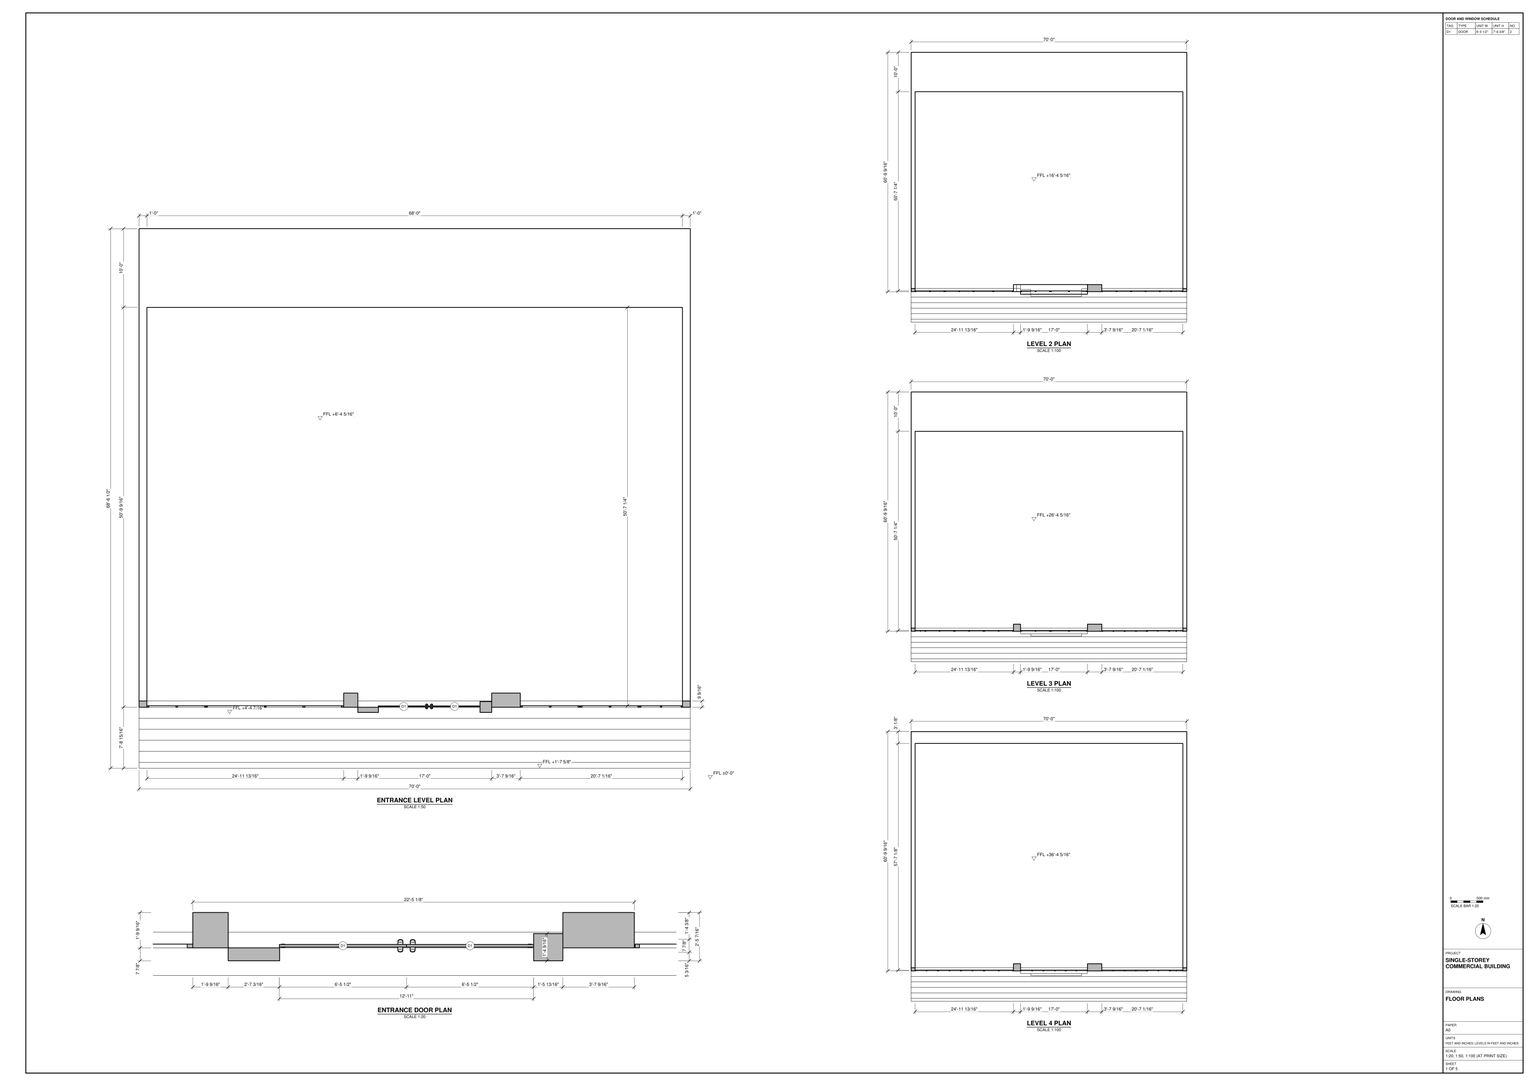
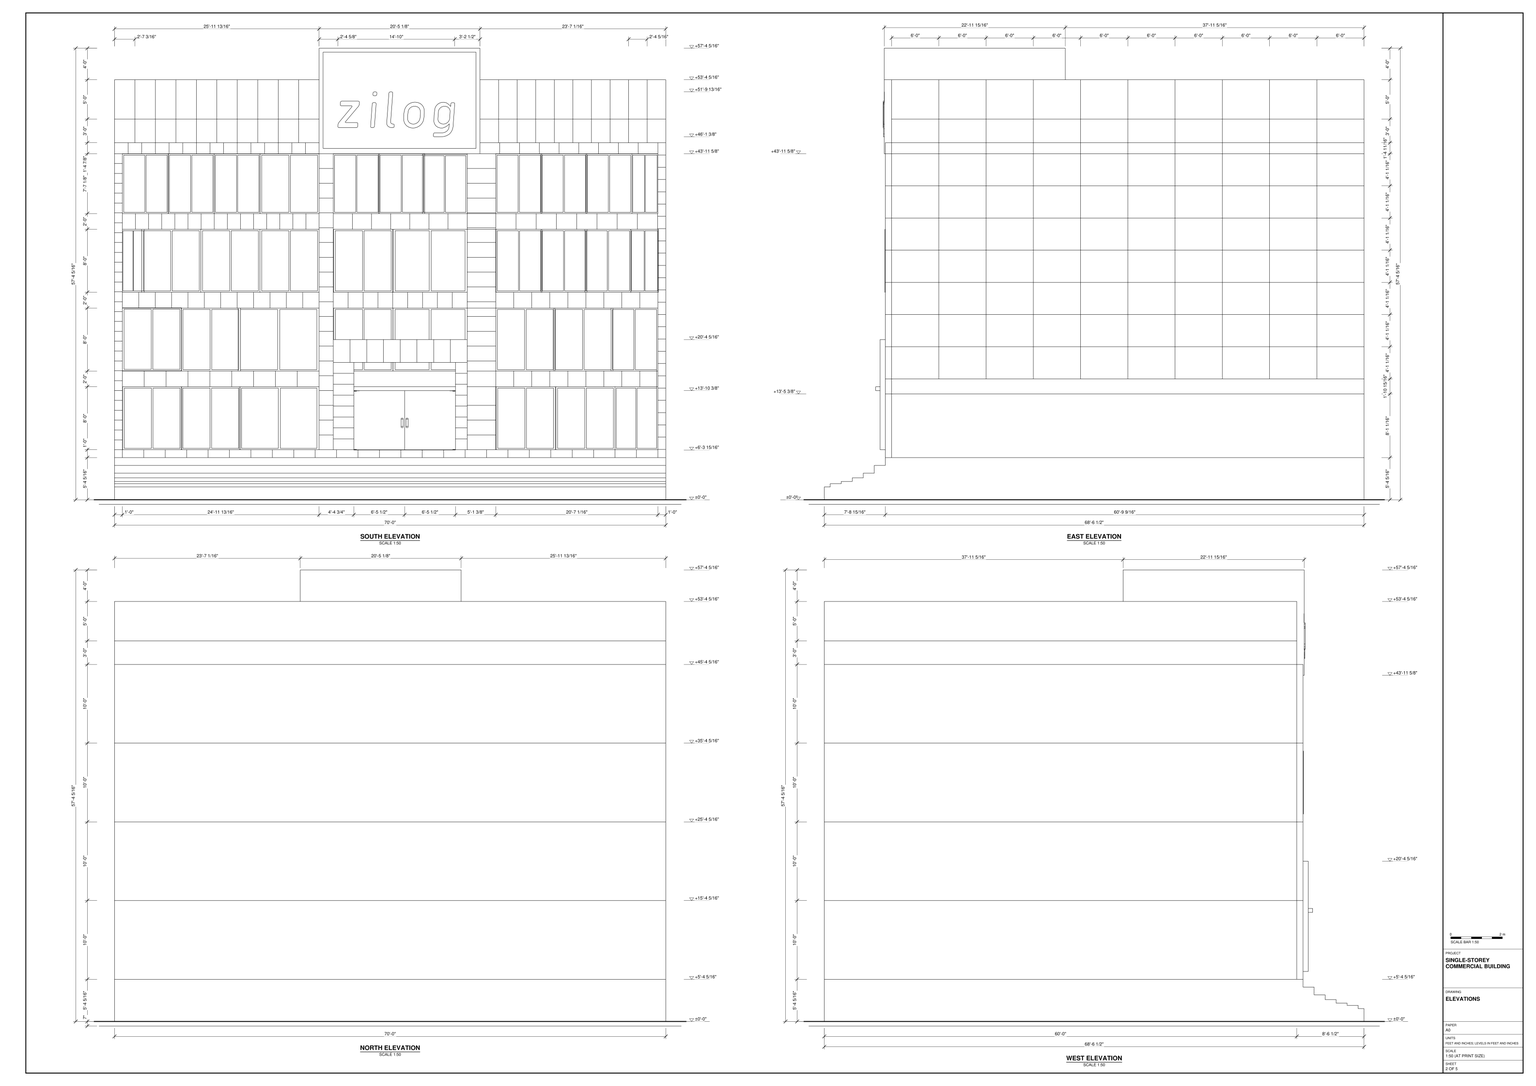
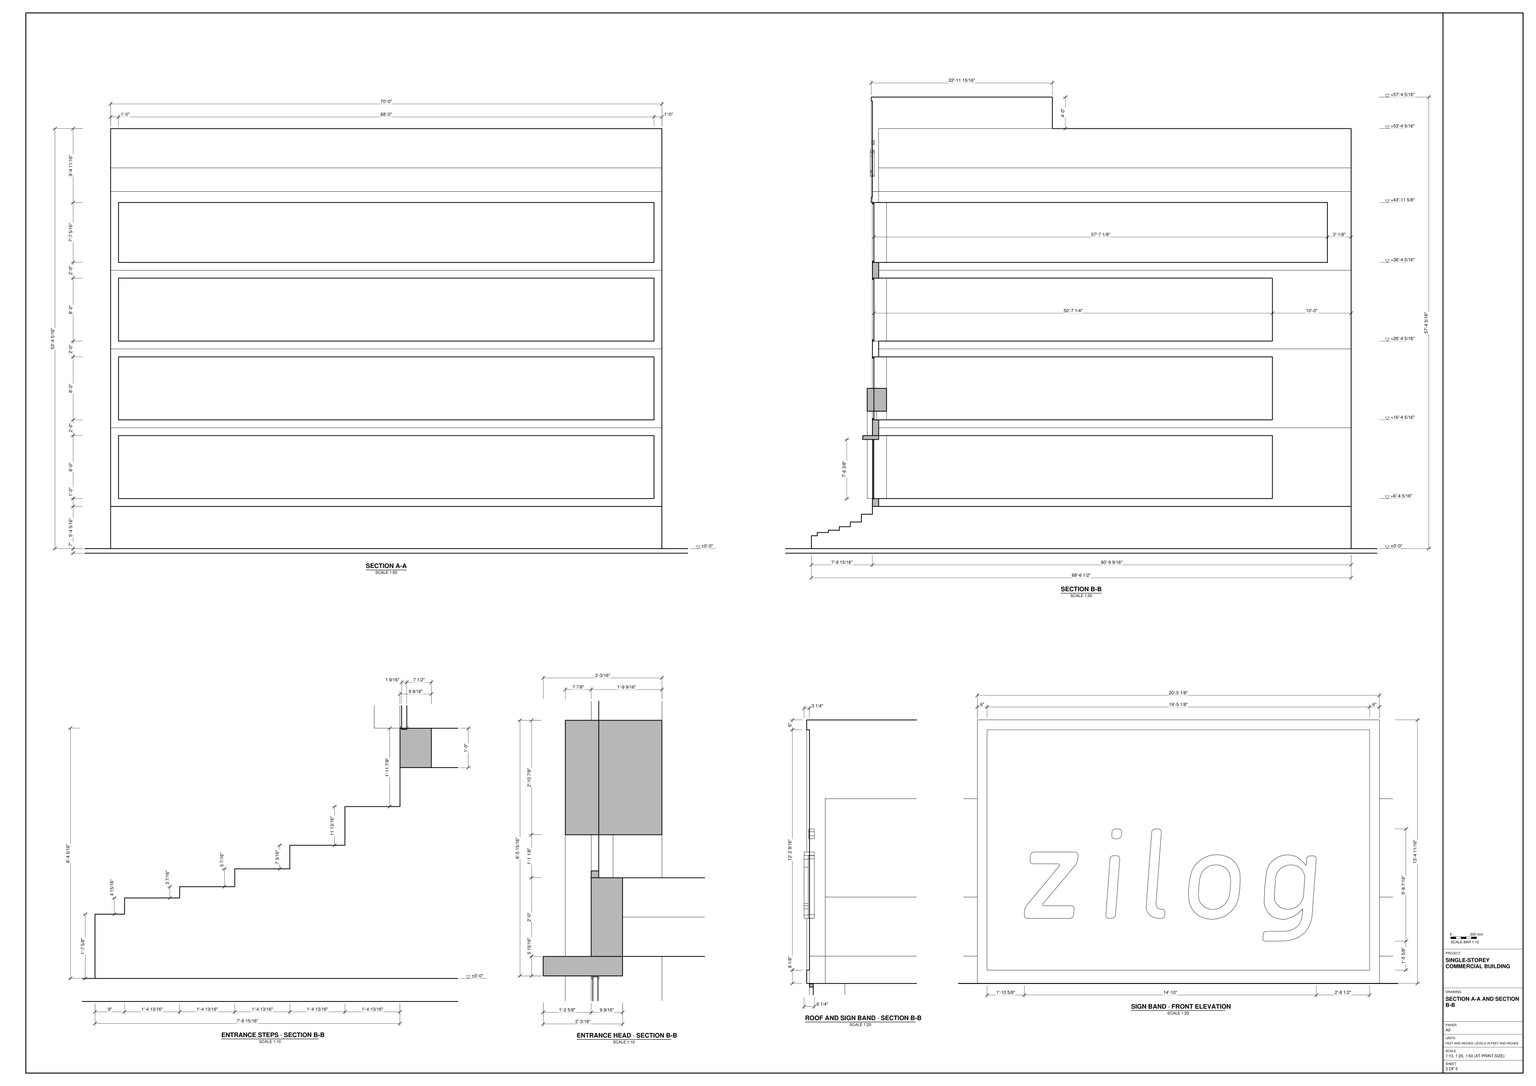
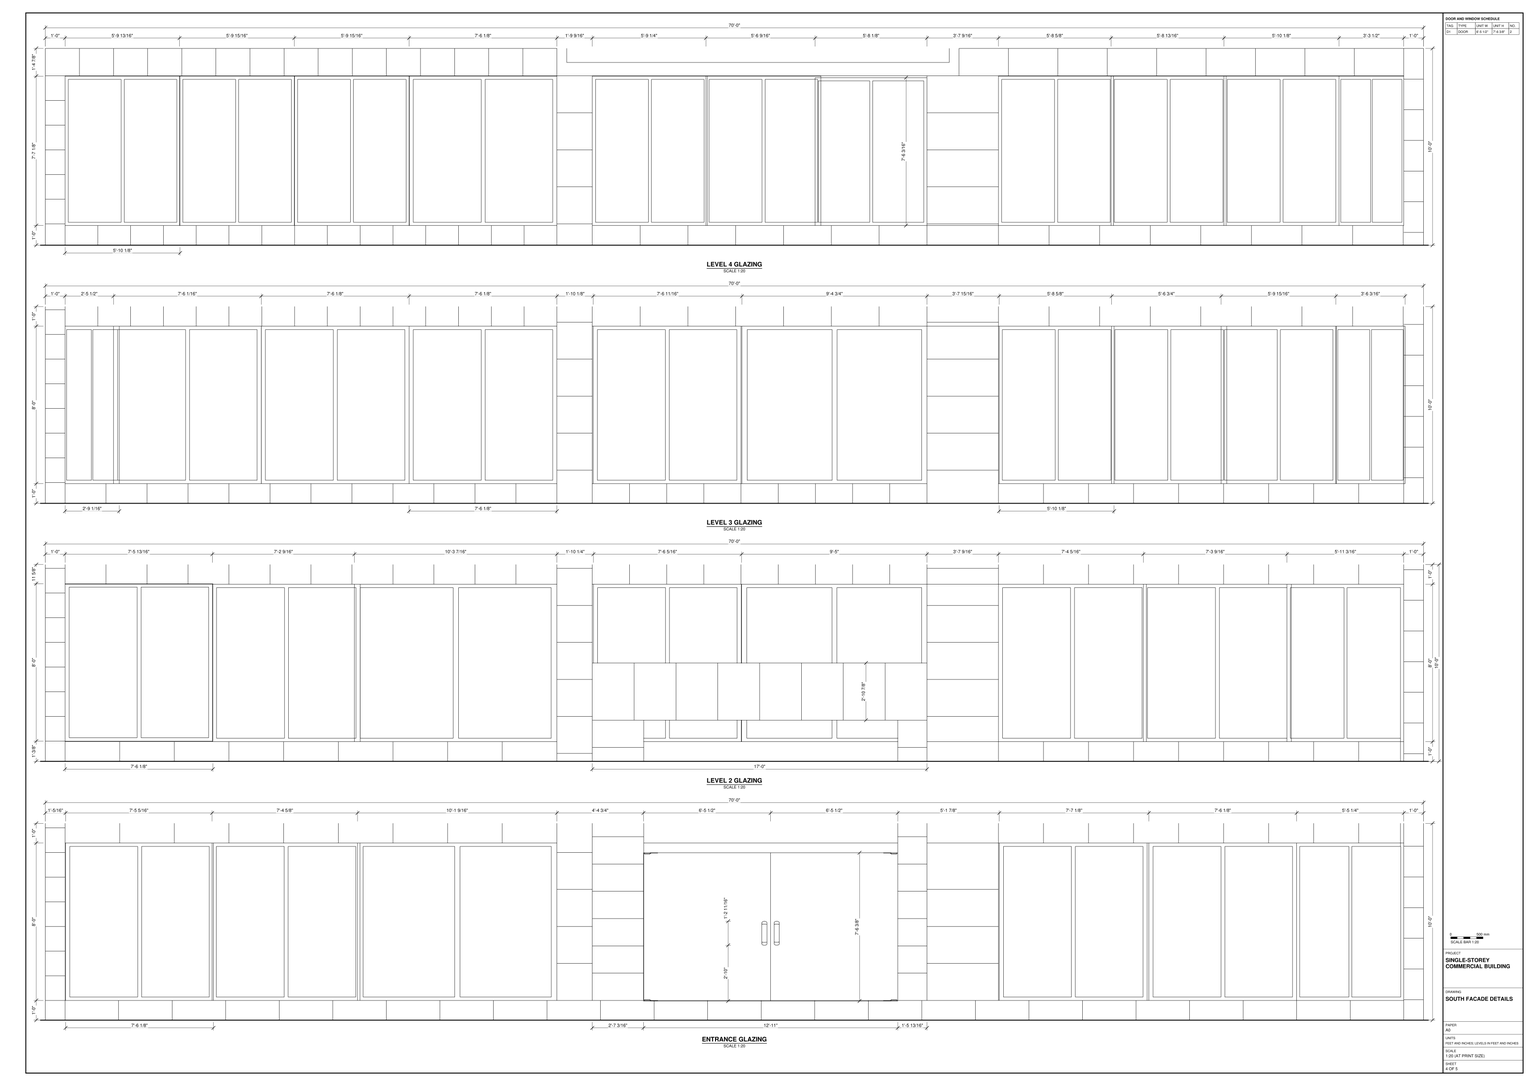
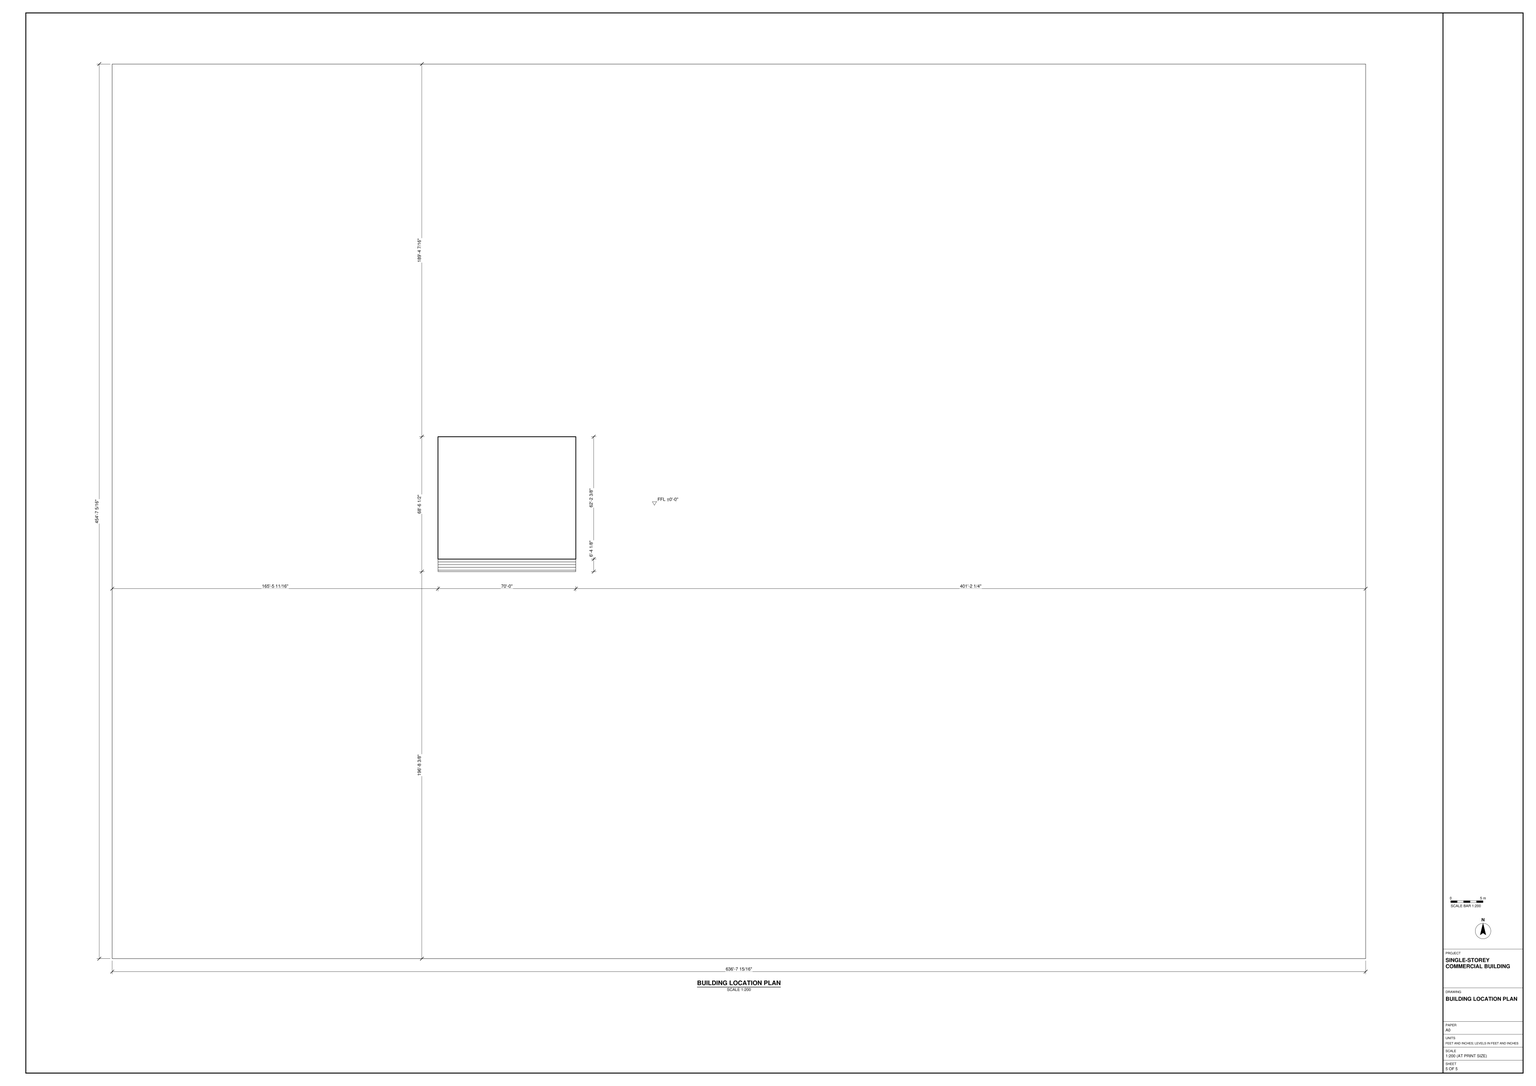
Build the commercial building in SketchUp from task_files/diagram_01.pdf. Work in feet and inches. The overall model extents are 636'-7 15/16" along X, 454'-7 5/16" along Y and 57'-11 5/16" along Z. These are the extents of the whole model; use the dimensioned plans for the building footprint. Set the ground datum at ±0'-0" and use the plans and sections to position the raised entrance floor and the three floors above it.

Model the rectangular shell with the wall and slab thicknesses shown in section. Keep the floor areas open and carry the uppermost floor space farther towards the rear than the spaces below it. Run the entrance steps across the south frontage to the paired glass doors. Use the entrance details to form the jambs and projecting head. Lay out the south window units in bays, matching the mullions and the bands between rows to the elevation. Distinguish the panel grid on the east wall from the horizontal divisions on the north and west walls. Finish the flat roof with the raised, framed sign panel above the entrance bay.

Make the walls, slabs and roof separate groups or components, and keep each furniture or joinery piece separate in the same way. Use components for repeated parts such as window units. Any decor or loose items shown may be represented by suitable library components. Save one SketchUp model as output_files/commercial_building_with_stepped_entrance_and_sign_band.skp.

# SketchUp Ruby script. Lengths in inches.
U = 1.inch
M = Sketchup.active_model
def pt(a) = Geom::Point3d.new(a.map { |v| v * U })
def face(e, loops, mat)
  f = e.add_face(loops[0].map { |a| pt(a) })
  loops[1..].each { |l| e.add_face(l.map { |a| pt(a) }).erase! }
  f.material = f.back_material = mat if mat
  f
end
# faces: each face lists its corners as indices into pts; further lists are holes
def faces(e, pts, list, mat = nil) = list.each { |f| face(e, (f[0].is_a?(Array) ? f : [f]).map { |l| l.map { |i| pts[i] } }, mat) }
# xy, xz, yz: faces in a plane at the given z, y or x. An outline is a flat list of corners, or four numbers for a rectangle; further outlines are holes
def ring(l) = l.size == 4 ? [[l[0], l[1]], [l[2], l[1]], [l[2], l[3]], [l[0], l[3]]] : l.each_slice(2).to_a
def flat(e, list, mat, &to3) = list.each { |f| face(e, (f[0].is_a?(Array) ? f : [f]).map { |l| ring(l).map { |u, v| to3.(u, v) } }, mat) }
def xy(e, z, list, mat = nil) = flat(e, list, mat) { |x, y| [x, y, z] }
def xz(e, y, list, mat = nil) = flat(e, list, mat) { |x, z| [x, y, z] }
def yz(e, x, list, mat = nil) = flat(e, list, mat) { |y, z| [x, y, z] }
def lines(e, pts, list) = list.each { |a, b| e.add_line(pt(pts[a]), pt(pts[b])) }
# prism: a flat outline (further loops are holes) pulled along v
def prism(e, loops, v, mat = nil)
  f = face(e, loops, mat); d = Geom::Vector3d.new(v.map { |x| x * U })
  f.pushpull(f.normal.samedirection?(d) ? d.length : -d.length)
end
def box(e, o, s, mat = nil) = prism(e, [[o, [o[0] + s[0], o[1], o[2]], [o[0] + s[0], o[1] + s[1], o[2]], [o[0], o[1] + s[1], o[2]]]], [0, 0, s[2]], mat)
def at(x, y, z, deg = 0) = Geom::Transformation.translation(pt([x, y, z])) * Geom::Transformation.rotation(ORIGIN, Z_AXIS, deg.degrees)
def axes(o, x, y, z) = Geom::Transformation.new([*x, 0, *y, 0, *z, 0, *pt(o).to_a, 1])
def part(name) = M.definitions.add(name)
# library, detail: a bought-in or finely detailed component or shape, given as its bounding box
def library(name, o, s) = part(name).tap { |d| box(d.entities, o, s) }
def detail(e, o, s) = box(e.add_group.entities, o, s)
def put(e, d, t, mat = nil) = e.add_instance(d, t).tap { |i| i.material = mat if mat }
def group(e, t, mat = nil) = e.add_group.tap { |g| g.transformation = t; g.material = mat if mat }.entities
root = M.entities
M.materials.add("2").color = [128, 128, 128]
M.materials["2"].alpha = 0.5
M.materials.add("Teddy_Shoes").color = [189, 191, 193]
M.materials.add("[0079_Teal]").color = [0, 68, 68]
M.materials.add("[0102_RoyalBlue]").color = [32, 52, 112]
M.materials.add("[0132_LightGray]").color = [169, 169, 169]
M.materials.add("[0134_DimGray]").color = [105, 105, 105]
M.materials.add("[0135_DarkGray]").color = [81, 81, 81]
M.materials.add("[0137_Black]").color = [0, 0, 0]
c1 = part("WindowDoubleBlack")
xy(c1.entities,0,[[0,0,96.0625,1.57]],"[0137_Black]")
xy(c1.entities,2.71,[[2.71,0,46.85,1.57],[49.41,0,93.35,1.57]],"[0137_Black]")
xy(c1.entities,122.09,[[2.71,0,46.85,1.57],[49.41,0,50,1.57],[50,0,93.35,1.57]],"[0137_Black]")
xy(c1.entities,124.8,[[0,0,96.0625,1.57]],"[0137_Black]")
xz(c1.entities,0,[[[0,0,96.0625,124.8],[2.71,2.71,46.85,122.09],[49.41,2.71,93.35,122.09]]],"[0137_Black]")
xz(c1.entities,1.57,[[2.71,2.71,46.85,122.09],[49.41,2.71,93.35,122.09]],"2")
xz(c1.entities,1.57,[[[0,0,96.0625,124.8],[2.71,2.71,46.85,122.09],[49.41,2.71,93.35,122.09]]],"[0137_Black]")
yz(c1.entities,0,[[0,0,1.57,124.8]],"[0137_Black]")
yz(c1.entities,2.71,[[0,2.71,1.57,122.09]],"[0137_Black]")
yz(c1.entities,46.85,[[0,2.71,1.57,122.09]],"[0137_Black]")
yz(c1.entities,49.41,[[0,2.71,1.57,122.09]],"[0137_Black]")
yz(c1.entities,93.35,[[0,2.71,1.57,122.09]],"[0137_Black]")
yz(c1.entities,96.0625,[[0,0,1.57,124.8]],"[0137_Black]")
c2 = library("Glass_door",[70.54,1.5625,0],[78.74,7.87,82.68])
c3 = library("Group\#1",[0,0,0],[237.3,8.35,91.24])
c4 = part("zilog")
put(c4.entities,c3,at(0,150.05,41.16))
xy(root,-25.25,[[0,0,7639.9375,5455.3125]])
xy(root,-18.22,[[[0,0,7639.9375,5455.3125],[1985.6875,2360.375,2825.6875,3182.875]],[1985.6875,2360.375,2825.6875,3182.875]])
xy(root,1.375,[[1985.6875,2360.375,2825.6875,2369.375]])
xy(root,6.3125,[[1985.6875,2369.375,2825.6875,2386.16]])
xy(root,9.75,[[1985.6875,2386.16,2825.6875,2402.95]])
xy(root,15.1875,[[1985.6875,2402.95,2825.6875,2419.74]])
xy(root,22.375,[[1985.6875,2419.74,2825.6875,2436.52]])
xy(root,34.1875,[[1985.6875,2436.52,2825.6875,2453.3125]])
xy(root,46.0625,[[1985.6875,2453.3125,2825.6875,2462.875],[1985.6875,2462.875,2825.6875,3182.875]],"[0102_RoyalBlue]")
xy(root,58.0625,[[2319.0625,2445.4375,2350.4375,2453.3125],[2505.24,2445.4375,2523.05,2453.3125],[1997.6875,2453.3125,2297.5,2462.875],[2297.5,2453.3125,2319.0625,2462.875],[2319.0625,2453.3125,2505.24,2453.3125,2505.24,2462,2523.05,2462,2523.05,2462.875,2319.0625,2462.875],
  [2505.24,2453.3125,2523.05,2462],[2523.05,2453.3125,2566.625,2462.875],[2566.625,2453.3125,2813.6875,2462.875],[1997.6875,2462.875,2297.5,2462.875,2297.5,2474.875,2319.0625,2474.875,2319.0625,2462.875,2523.05,2462.875,2523.05,2474.875,2566.625,2474.875,2566.625,2462.875,2813.6875,2462.875,2813.6875,3062.875,1997.6875,3062.875],[2297.5,2462.875,2319.0625,2474.875],
  [2523.05,2462.875,2566.625,2474.875]],"[0102_RoyalBlue]")
xy(root,148.125,[[2350.4375,2438.6875,2350.4375,2453.3125,2319.0625,2453.3125,2319.0625,2462.875,2505.24,2462.875,2505.24,2438.6875]],"[0102_RoyalBlue]")
xy(root,154.0625,[[2350.4375,2438.6875,2505.24,2453.3125],[1997.6875,2453.3125,2297.5,2462.875],[2319.0625,2453.3125,2505.24,2462.875],[2505.24,2453.3125,2813.6875,2462.875],[1997.6875,2462.875,1997.6875,3062.875,2813.6875,3062.875,2813.6875,2462.875,2566.625,2462.875,2566.625,2474.875,2523.05,2474.875,2523.05,2462.875,2319.0625,2462.875,2319.0625,2474.875,2297.5,2474.875,2297.5,2462.875],
  [2297.5,2462.875,2307.0625,2474.875],[2307.0625,2462.875,2319.0625,2474.875],[2523.05,2462.875,2566.625,2474.875]],"[0102_RoyalBlue]")
xy(root,178.0625,[[1997.6875,2453.3125,2297.5,2462.875],[2319.0625,2453.3125,2350.4375,2459.9375],[2350.4375,2453.3125,2813.6875,2453.3125,2813.6875,2462.875,2319.0625,2462.875,2319.0625,2459.9375,2350.4375,2459.9375],[1997.6875,2462.875,2297.5,2462.875,2297.5,2474.875,2319.0625,2474.875,2319.0625,2462.875,2523.05,2462.875,2523.05,2474.875,2566.625,2474.875,2566.625,2462.875,2813.6875,2462.875,2813.6875,3062.875,1997.6875,3062.875],[2297.5,2462.875,2307.0625,2474.875],
  [2307.0625,2462.875,2319.0625,2474.875],[2523.05,2462.875,2566.625,2474.875]],"[0102_RoyalBlue]")
xy(root,191.17,[[2350.4375,2445.4375,2350.4375,2459.9375,2319.0625,2459.9375,2319.0625,2474.875,2523.05,2474.875,2523.05,2462,2505.24,2462,2505.24,2445.4375]],"[0102_RoyalBlue]")
xy(root,226.0625,[[2319.0625,2445.4375,2523.05,2474.875]],"[0134_DimGray]")
xy(root,274.0625,[[1997.6875,2453.3125,2297.5,2462.875],[2319.0625,2453.3125,2813.6875,2462.875],[1997.6875,2462.875,1997.6875,3062.875,2813.6875,3062.875,2813.6875,2462.875,2566.625,2462.875,2566.625,2474.875,2523.05,2474.875,2523.05,2462.875,2319.0625,2462.875,2319.0625,2474.875,2297.5,2474.875,2297.5,2462.875],[2297.5,2462.875,2307.0625,2474.875],[2307.0625,2462.875,2319.0625,2474.875],
  [2523.05,2462.875,2566.625,2474.875]],"[0102_RoyalBlue]")
xy(root,298.0625,[[1997.6875,2453.3125,2297.5,2462.875],[1997.6875,2462.875,2297.5,2462.875,2297.5,2474.875,2319.0625,2474.875,2319.0625,2462.875,2523.05,2462.875,2523.05,2474.875,2566.625,2474.875,2566.625,2462.875,2813.6875,2462.875,2813.6875,3062.875,1997.6875,3062.875],[2297.5,2462.875,2307.0625,2474.875],[2307.0625,2462.875,2319.0625,2474.875],[2523.05,2462.875,2566.625,2474.875]],"[0102_RoyalBlue]")
xy(root,394.0625,[[1997.6875,2453.3125,2297.5,2462.875],[2319.0625,2453.3125,2813.6875,2462.875],[1997.6875,2462.875,1997.6875,3062.875,2813.6875,3062.875,2813.6875,2462.875,2566.625,2462.875,2566.625,2474.875,2523.05,2474.875,2523.05,2462.875,2319.0625,2462.875,2319.0625,2474.875,2297.5,2474.875,2297.5,2462.875],[2297.5,2462.875,2307.0625,2474.875],[2307.0625,2462.875,2319.0625,2474.875],
  [2523.05,2462.875,2566.625,2474.875]],"[0102_RoyalBlue]")
xy(root,418.0625,[[1997.6875,2453.3125,2297.5,2462.875],[2319.0625,2453.3125,2813.6875,2462.875],[1997.6875,2462.875,2297.5,2462.875,2297.5,2474.875,2319.0625,2474.875,2319.0625,2462.875,2523.05,2462.875,2523.05,2474.875,2566.625,2474.875,2566.625,2462.875,2813.6875,2462.875,2813.6875,3146.75,1997.6875,3146.75],[2297.5,2462.875,2307.0625,2474.875],[2307.0625,2462.875,2319.0625,2474.875],
  [2523.05,2462.875,2566.625,2474.875]],"[0102_RoyalBlue]")
xy(root,509.375,[[2297.5,2451.625,2542.625,2453.3125],[1997.6875,2453.3125,2297.5,2462.875],[2297.5,2453.3125,2319.0625,2474.875],[2319.0625,2453.3125,2523.05,2462.875],[2523.05,2453.3125,2542.625,2474.875],
  [2542.625,2453.3125,2566.625,2462.875],[2566.625,2453.3125,2813.6875,2462.875],[1997.6875,2462.875,1997.6875,3146.75,2813.6875,3146.75,2813.6875,2462.875,2566.625,2462.875,2566.625,2474.875,2523.05,2474.875,2523.05,2462.875,2319.0625,2462.875,2319.0625,2474.875,2297.5,2474.875,2297.5,2462.875],[2542.625,2462.875,2566.625,2474.875]],"[0102_RoyalBlue]")
xy(root,517.5,[[2303.5,2451.625,2536.625,2453.3125]],"[0102_RoyalBlue]")
xy(root,526.0625,[[1985.6875,2453.3125,2297.5,2462.875],[2542.625,2453.3125,2825.6875,2462.875]],"[0102_RoyalBlue]")
xy(root,622.0625,[[1985.6875,2462.875,2297.5,3182.875],[2542.625,2462.875,2825.6875,3182.875],[2297.5,2727.59,2542.625,3182.875]],"[0102_RoyalBlue]")
xy(root,664.0625,[[2303.5,2451.625,2536.625,2453.3125]])
xy(root,670.0625,[[2297.5,2451.625,2542.625,2727.59]],"[0102_RoyalBlue]")
xz(root,0,[[0,-25.25,7639.9375,-18.22]])
xz(root,2360.375,[[1985.6875,-18.22,2825.6875,1.375]])
xz(root,2369.375,[[1985.6875,1.375,2825.6875,6.3125]])
xz(root,2386.16,[[1985.6875,6.3125,2825.6875,9.75]])
xz(root,2402.95,[[1985.6875,9.75,2825.6875,15.1875]])
xz(root,2419.74,[[1985.6875,15.1875,2825.6875,22.375]])
xz(root,2436.52,[[1985.6875,22.375,2825.6875,34.1875]])
xz(root,2438.6875,[[2350.4375,148.125,2505.24,154.0625]],"[0102_RoyalBlue]")
xz(root,2445.4375,[[2319.0625,58.0625,2350.4375,74.7],[2505.24,58.0625,2523.05,74.7],[2319.0625,74.7,2350.4375,91.34],[2505.24,74.7,2523.05,91.34],[2319.0625,91.34,2350.4375,107.98],
  [2505.24,91.34,2523.05,107.98],[2319.0625,107.98,2350.4375,124.62],[2505.24,107.98,2523.05,124.62],[2319.0625,124.62,2350.4375,141.26],[2505.24,124.62,2523.05,141.26],
  [2319.0625,141.26,2350.4375,157.9],[2505.24,141.26,2523.05,157.9],[2319.0625,157.9,2350.4375,174.53],[2505.24,157.9,2523.05,174.53],[2319.0625,174.53,2350.4375,191.17],
  [2505.24,174.53,2523.05,191.17],[2319.0625,191.17,2344.5625,226.0625],[2344.5625,191.17,2370.06,226.0625],[2370.06,191.17,2395.56,226.0625],[2395.56,191.17,2421.06,226.0625],
  [2421.06,191.17,2446.56,226.0625],[2446.56,191.17,2472.05,226.0625],[2472.05,191.17,2497.55,226.0625],[2497.55,191.17,2523.05,226.0625]],"[0134_DimGray]")
xz(root,2451.625,[[[2297.5,509.375,2542.625,670.0625],[2303.5,517.5,2536.625,664.0625]]],"[0102_RoyalBlue]")
xz(root,2453.3125,[[1985.6875,34.1875,2825.6875,46.0625]])
xz(root,2453.3125,[[2519.93,46.0625,2552.57,58.0625],[2552.57,46.0625,2585.21,58.0625],[2585.21,46.0625,2617.85,58.0625],[2617.85,46.0625,2650.49,58.0625],[2650.49,46.0625,2683.13,58.0625],
  [2683.13,46.0625,2715.77,58.0625],[2715.77,46.0625,2748.41,58.0625],[2748.41,46.0625,2781.05,58.0625],[2781.05,46.0625,2813.6875,58.0625],[2813.6875,46.0625,2825.6875,58.5625],
  [2813.6875,58.5625,2825.6875,77.26],[2813.6875,77.26,2825.6875,95.96],[2813.6875,95.96,2825.6875,114.66],[2813.6875,114.66,2825.6875,133.36],[2813.6875,133.36,2825.6875,152.0625],
  [2813.6875,152.0625,2825.6875,170.76],[2566.625,154.0625,2594.08,178.0625],[2594.08,154.0625,2621.53,178.0625],[2621.53,154.0625,2648.98,178.0625],[2648.98,154.0625,2676.43,178.0625],
  [2676.43,154.0625,2703.88,178.0625],[2703.88,154.0625,2731.33,178.0625],[2731.33,154.0625,2758.78,178.0625],[2758.78,154.0625,2786.24,178.0625],[2786.24,154.0625,2811.68,178.0625],
  [1997.6875,274.0625,2022.67,298.0625],[2022.67,274.0625,2047.66,298.0625],[2047.66,274.0625,2072.64,298.0625],[2072.64,274.0625,2097.625,298.0625],[2097.625,274.0625,2122.61,298.0625],
  [2122.61,274.0625,2147.59,298.0625],[2147.59,274.0625,2172.58,298.0625],[2172.58,274.0625,2197.5625,298.0625],[2197.5625,274.0625,2222.55,298.0625],[2222.55,274.0625,2247.53,298.0625],
  [2247.53,274.0625,2272.52,298.0625],[2272.52,274.0625,2297.5,298.0625],[2319.0625,394.0625,2348.2,418.0625],[2348.2,394.0625,2377.35,418.0625],[2377.35,394.0625,2406.49,418.0625],
  [2406.49,394.0625,2435.63,418.0625],[2435.63,394.0625,2464.77,418.0625],[2464.77,394.0625,2493.91,418.0625],[2493.91,394.0625,2523.05,418.0625],[2813.6875,469.96,2825.6875,488.66],
  [2813.6875,488.66,2825.6875,507.36],[2813.6875,507.36,2825.6875,526.0625],[2542.625,509.375,2572.74,526.0625],[2572.74,509.375,2602.86,526.0625],[2602.86,509.375,2632.98,526.0625],
  [2632.98,509.375,2663.1,526.0625],[2663.1,509.375,2693.22,526.0625],[2693.22,509.375,2723.33,526.0625],[2723.33,509.375,2753.45,526.0625],[2753.45,509.375,2783.57,526.0625],
  [2783.57,509.375,2813.6875,526.0625]],"Teddy_Shoes")
xz(root,2453.3125,[[1985.6875,46.0625,1997.6875,58.0625],[1997.6875,46.0625,2030.33,58.0625],[2030.33,46.0625,2062.97,58.0625],[2062.97,46.0625,2095.61,58.0625],[2095.61,46.0625,2128.25,58.0625],
  [2128.25,46.0625,2160.89,58.0625],[2160.89,46.0625,2193.53,58.0625],[2193.53,46.0625,2226.17,58.0625],[2226.17,46.0625,2258.81,58.0625],[2258.81,46.0625,2291.45,58.0625],
  [2291.45,46.0625,2324.09,58.0625],[2324.09,46.0625,2356.73,58.0625],[2356.73,46.0625,2389.37,58.0625],[2389.37,46.0625,2422.01,58.0625],[2422.01,46.0625,2454.65,58.0625],
  [2454.65,46.0625,2487.29,58.0625],[2487.29,46.0625,2519.93,58.0625],[1985.6875,58.0625,1997.6875,73.11],[2297.5,58.0625,2319.0625,80.63],[2319.0625,58.0625,2350.4375,148.125],
  [2523.05,58.0625,2566.625,80.63],[1985.6875,73.11,1997.6875,88.15],[2297.5,80.63,2319.0625,103.19],[2523.05,80.63,2566.625,103.19],[1985.6875,88.15,1997.6875,103.19],
  [1985.6875,103.19,1997.6875,118.24],[2297.5,103.19,2319.0625,125.76],[2523.05,103.19,2566.625,125.76],[1985.6875,118.24,1997.6875,133.28],[2297.5,125.76,2319.0625,148.32],
  [2523.05,125.76,2566.625,154.0625],[1985.6875,133.28,1997.6875,148.33],[2319.0625,148.125,2350.4375,154.0625],[2297.5,148.32,2319.0625,170.89],[1985.6875,148.33,1997.6875,163.37],
  [1997.6875,154.0625,2031,178.0625],[2031,154.0625,2064.3125,178.0625],[2064.3125,154.0625,2097.625,178.0625],[2097.625,154.0625,2130.9375,178.0625],[2130.9375,154.0625,2164.25,178.0625],
  [2164.25,154.0625,2197.5625,178.0625],[2197.5625,154.0625,2230.875,178.0625],[2230.875,154.0625,2264.1875,178.0625],[2264.1875,154.0625,2297.5,178.0625],[2319.0625,154.0625,2350.4375,178.0625],
  [2350.4375,154.0625,2523.05,178.0625],[2523.05,154.0625,2566.625,178.0625],[2811.68,154.0625,2813.6875,178.0625],[1985.6875,163.37,1997.6875,178.41],[2813.6875,170.76,2825.6875,189.46],
  [2297.5,170.89,2319.0625,193.46],[2523.05,178.0625,2566.625,193.46],[1985.6875,178.41,1997.6875,193.46],[2813.6875,189.46,2825.6875,208.16],[1985.6875,193.46,1997.6875,208.5],
  [2297.5,193.46,2319.0625,216.02],[2523.05,193.46,2566.625,216.02],[2813.6875,208.16,2825.6875,226.86],[1985.6875,208.5,1997.6875,223.54],[2297.5,216.02,2319.0625,238.59],
  [2523.05,216.02,2566.625,238.59],[1985.6875,223.54,1997.6875,238.59],[2813.6875,226.86,2825.6875,245.5625],[1985.6875,238.59,1997.6875,253.63],[2297.5,238.59,2319.0625,261.15],
  [2523.05,238.59,2566.625,261.15],[2813.6875,245.5625,2825.6875,264.26],[1985.6875,253.63,1997.6875,268.68],[2297.5,261.15,2319.0625,283.72],[2523.05,261.15,2566.625,274.0625],
  [2813.6875,264.26,2825.6875,282.96],[1985.6875,268.68,1997.6875,283.72],[2319.0625,274.0625,2341.73,298.0625],[2341.73,274.0625,2364.39,298.0625],[2364.39,274.0625,2387.06,298.0625],
  [2387.06,274.0625,2409.72,298.0625],[2409.72,274.0625,2432.39,298.0625],[2432.39,274.0625,2455.06,298.0625],[2455.06,274.0625,2477.72,298.0625],[2477.72,274.0625,2500.39,298.0625],
  [2500.39,274.0625,2523.05,298.0625],[2523.05,274.0625,2566.625,283.72],[2813.6875,282.96,2825.6875,301.66],[1985.6875,283.72,1997.6875,298.76],[2297.5,283.72,2319.0625,306.28],
  [2523.05,283.72,2566.625,306.28],[1985.6875,298.76,1997.6875,313.81],[2813.6875,301.66,2825.6875,320.36],[2297.5,306.28,2319.0625,328.85],[2523.05,306.28,2566.625,328.85],
  [1985.6875,313.81,1997.6875,328.85],[2813.6875,320.36,2825.6875,339.0625],[1985.6875,328.85,1997.6875,343.89],[2297.5,328.85,2319.0625,351.42],[2523.05,328.85,2566.625,351.42],
  [2813.6875,339.0625,2825.6875,357.76],[1985.6875,343.89,1997.6875,358.9375],[2297.5,351.42,2319.0625,373.98],[2523.05,351.42,2566.625,373.98],[2813.6875,357.76,2825.6875,376.46],
  [1985.6875,358.9375,1997.6875,373.98],[1985.6875,373.98,1997.6875,389.02],[2297.5,373.98,2319.0625,396.55],[2523.05,373.98,2566.625,394.0625],[2813.6875,376.46,2825.6875,376.46,2825.6875,432.5625,2813.6875,432.5625,2813.6875,418.0625,2813.3125,418.0625,2813.3125,394.0625,2813.6875,394.0625],
  [1985.6875,389.02,1997.6875,404.07],[2523.05,394.0625,2566.625,396.55],[2297.5,396.55,2319.0625,419.11],[2523.05,396.55,2566.625,418.0625],[1985.6875,404.07,1997.6875,419.11],
  [2523.05,418.0625,2566.625,419.11],[1985.6875,419.11,1997.6875,434.16],[2297.5,419.11,2319.0625,441.68],[2523.05,419.11,2566.625,441.68],[2813.6875,432.5625,2825.6875,451.26],
  [1985.6875,434.16,1997.6875,449.2],[2297.5,441.68,2319.0625,464.24],[2523.05,441.68,2566.625,464.24],[1985.6875,449.2,1997.6875,464.24],[2813.6875,451.26,2825.6875,469.96],
  [1985.6875,464.24,1997.6875,479.29],[2297.5,464.24,2319.0625,486.81],[2523.05,464.24,2566.625,486.81],[1985.6875,479.29,1997.6875,494.33],[2297.5,486.81,2319.0625,509.375],
  [2523.05,486.81,2566.625,509.375],[1985.6875,494.33,1997.6875,509.375],[1985.6875,509.375,2006.48,526.0625],[2006.48,509.375,2027.26,526.0625],[2027.26,509.375,2048.05,526.0625],
  [2048.05,509.375,2068.84,526.0625],[2068.84,509.375,2089.625,526.0625],[2089.625,509.375,2110.41,526.0625],[2110.41,509.375,2131.2,526.0625],[2131.2,509.375,2151.99,526.0625],
  [2151.99,509.375,2172.78,526.0625],[2172.78,509.375,2193.5625,526.0625],[2193.5625,509.375,2214.35,526.0625],[2214.35,509.375,2235.14,526.0625],[2235.14,509.375,2255.93,526.0625],
  [2255.93,509.375,2276.71,526.0625],[2276.71,509.375,2297.5,526.0625],[2303.5,517.5,2536.625,664.0625]],"[0102_RoyalBlue]")
xz(root,2453.3125,[[2566.625,274.0625,2594.08,298.0625],[2594.08,274.0625,2621.53,298.0625],[2621.53,274.0625,2648.98,298.0625],[2648.98,274.0625,2676.43,298.0625],[2676.43,274.0625,2703.88,298.0625],
  [2703.88,274.0625,2731.33,298.0625],[2731.33,274.0625,2758.78,298.0625],[2758.78,274.0625,2786.24,298.0625],[2786.24,274.0625,2813.6875,298.0625],[1997.6875,394.0625,2017.68,418.0625],
  [2017.68,394.0625,2037.66,418.0625],[2037.66,394.0625,2057.65,418.0625],[2057.65,394.0625,2077.64,418.0625],[2077.64,394.0625,2097.625,418.0625],[2097.625,394.0625,2117.61,418.0625],
  [2117.61,394.0625,2137.6,418.0625],[2137.6,394.0625,2157.59,418.0625],[2157.59,394.0625,2177.57,418.0625],[2177.57,394.0625,2197.5625,418.0625],[2197.5625,394.0625,2217.55,418.0625],
  [2217.55,394.0625,2237.54,418.0625],[2237.54,394.0625,2257.52,418.0625],[2257.52,394.0625,2277.51,418.0625],[2277.51,394.0625,2297.5,418.0625],[2566.625,394.0625,2597.46,418.0625],
  [2597.46,394.0625,2628.3,418.0625],[2628.3,394.0625,2659.13,418.0625],[2659.13,394.0625,2689.97,418.0625],[2689.97,394.0625,2720.8,418.0625],[2720.8,394.0625,2751.64,418.0625],
  [2751.64,394.0625,2782.48,418.0625],[2782.48,394.0625,2813.3125,418.0625]],"[0134_DimGray]")
xz(root,2459.9375,[[2319.0625,178.0625,2350.4375,191.17]],"[0102_RoyalBlue]")
xz(root,2462,[[2505.24,58.0625,2523.05,191.17]],"[0102_RoyalBlue]")
xz(root,2462.875,[[1985.6875,526.0625,2016.87,562.0625],[2016.87,526.0625,2048.05,562.0625],[2048.05,526.0625,2079.23,562.0625],[2079.23,526.0625,2110.41,562.0625],[2110.41,526.0625,2141.59,562.0625],
  [2141.59,526.0625,2172.78,562.0625],[2172.78,526.0625,2203.96,562.0625],[2203.96,526.0625,2235.14,562.0625],[2235.14,526.0625,2266.32,562.0625],[2266.32,526.0625,2297.5,562.0625],
  [2542.625,526.0625,2570.93,562.0625],[2570.93,526.0625,2599.24,562.0625],[2599.24,526.0625,2627.54,562.0625],[2627.54,526.0625,2655.85,562.0625],[2655.85,526.0625,2684.16,562.0625],
  [2684.16,526.0625,2712.46,562.0625],[2712.46,526.0625,2740.77,562.0625],[2740.77,526.0625,2769.08,562.0625],[2769.08,526.0625,2797.38,562.0625],[2797.38,526.0625,2825.6875,562.0625]],"Teddy_Shoes")
xz(root,2462.875,[[1985.6875,46.0625,1985.6875,526.0625,2297.5,526.0625,2297.5,509.375,1997.6875,509.375,1997.6875,418.0625,2297.5,418.0625,2297.5,394.0625,1997.6875,394.0625,1997.6875,298.0625,2297.5,298.0625,2297.5,274.0625,1997.6875,274.0625,1997.6875,178.0625,2297.5,178.0625,2297.5,154.0625,1997.6875,154.0625,1997.6875,58.0625,2813.6875,58.0625,2813.6875,154.0625,2566.625,154.0625,2566.625,178.0625,2813.6875,178.0625,2813.6875,274.0625,2566.625,274.0625,2566.625,298.0625,2813.6875,298.0625,2813.6875,394.0625,2566.625,394.0625,2566.625,418.0625,2813.6875,418.0625,2813.6875,509.375,2542.625,509.375,2542.625,526.0625,2825.6875,526.0625,2825.6875,46.0625],[2319.0625,148.125,2505.24,154.0625],[2297.5,154.0625,2307.0625,178.0625],[2307.0625,154.0625,2523.05,178.0625],[2523.05,154.0625,2566.625,178.0625],
  [2297.5,274.0625,2307.0625,298.0625],[2307.0625,274.0625,2523.05,298.0625],[2523.05,274.0625,2566.625,298.0625],[2297.5,394.0625,2307.0625,418.0625],[2307.0625,394.0625,2523.05,418.0625],
  [2523.05,394.0625,2566.625,418.0625]],"[0102_RoyalBlue]")
xz(root,2462.875,[[1985.6875,562.0625,2016.87,622.0625],[2016.87,562.0625,2048.05,622.0625],[2048.05,562.0625,2079.23,622.0625],[2079.23,562.0625,2110.41,622.0625],[2110.41,562.0625,2141.59,622.0625],
  [2141.59,562.0625,2172.78,622.0625],[2172.78,562.0625,2203.96,622.0625],[2203.96,562.0625,2235.14,622.0625],[2235.14,562.0625,2266.32,622.0625],[2266.32,562.0625,2297.5,622.0625],
  [2542.625,562.0625,2570.93,622.0625],[2570.93,562.0625,2599.24,622.0625],[2599.24,562.0625,2627.54,622.0625],[2627.54,562.0625,2655.85,622.0625],[2655.85,562.0625,2684.16,622.0625],
  [2684.16,562.0625,2712.46,622.0625],[2712.46,562.0625,2740.77,622.0625],[2740.77,562.0625,2769.08,622.0625],[2769.08,562.0625,2797.38,622.0625],[2797.38,562.0625,2825.6875,622.0625]],"[0134_DimGray]")
xz(root,2474.875,[[2297.5,58.0625,2319.0625,154.0625],[2523.05,58.0625,2566.625,154.0625],[2297.5,178.0625,2297.5,274.0625,2319.0625,274.0625,2319.0625,226.0625,2523.05,226.0625,2523.05,191.17,2319.0625,191.17,2319.0625,178.0625],[2523.05,178.0625,2566.625,274.0625],[2297.5,298.0625,2319.0625,394.0625],
  [2523.05,298.0625,2566.625,394.0625],[2297.5,418.0625,2319.0625,509.375],[2523.05,418.0625,2566.625,509.375]],"[0102_RoyalBlue]")
xz(root,2727.59,[[2297.5,622.0625,2542.625,670.0625]],"[0102_RoyalBlue]")
xz(root,3062.875,[[1997.6875,58.0625,2813.6875,154.0625],[1997.6875,178.0625,2813.6875,274.0625],[1997.6875,298.0625,2813.6875,394.0625]],"[0102_RoyalBlue]")
xz(root,3146.75,[[1997.6875,418.0625,2813.6875,509.375]],"[0102_RoyalBlue]")
xz(root,3182.875,[[1985.6875,-18.22,2825.6875,46.0625]])
xz(root,3182.875,[[1985.6875,46.0625,2825.6875,166.0625],[1985.6875,166.0625,2825.6875,286.0625],[1985.6875,286.0625,2825.6875,406.0625],[1985.6875,406.0625,2825.6875,526.0625],[1985.6875,526.0625,2825.6875,562.0625],
  [1985.6875,562.0625,2825.6875,622.0625]],"[0102_RoyalBlue]")
xz(root,5455.3125,[[0,-25.25,7639.9375,-18.22]])
yz(root,0,[[0,-25.25,5455.3125,-18.22]])
yz(root,1985.6875,[[2360.375,-18.22,2360.375,1.375,2369.375,1.375,2369.375,6.3125,2386.16,6.3125,2386.16,9.75,2402.95,9.75,2402.95,15.1875,2419.74,15.1875,2419.74,22.375,2436.52,22.375,2436.52,34.1875,2453.3125,34.1875,2453.3125,46.0625,3182.875,46.0625,3182.875,-18.22]])
yz(root,1985.6875,[[2453.3125,46.0625,2462.875,166.0625],[2462.875,46.0625,3182.875,166.0625],[2453.3125,166.0625,2462.875,286.0625],[2462.875,166.0625,3182.875,286.0625],[2453.3125,286.0625,2462.875,406.0625],
  [2462.875,286.0625,3182.875,406.0625],[2453.3125,406.0625,2462.875,526.0625],[2462.875,406.0625,3182.875,526.0625],[2462.875,526.0625,3182.875,562.0625],[2462.875,562.0625,3182.875,622.0625]],"[0102_RoyalBlue]")
yz(root,1997.6875,[[2453.3125,58.0625,2462.875,154.0625],[2462.875,58.0625,3062.875,154.0625],[2453.3125,178.0625,2462.875,274.0625],[2462.875,178.0625,3062.875,274.0625],[2453.3125,298.0625,2462.875,394.0625],
  [2462.875,298.0625,3062.875,394.0625],[2453.3125,418.0625,2462.875,509.375],[2462.875,418.0625,3146.75,509.375]],"[0102_RoyalBlue]")
yz(root,2297.5,[[2453.3125,58.0625,2474.875,154.0625],[2453.3125,154.0625,2462.875,178.0625],[2453.3125,178.0625,2474.875,274.0625],[2453.3125,274.0625,2462.875,298.0625],[2453.3125,298.0625,2474.875,394.0625],
  [2453.3125,394.0625,2462.875,418.0625],[2453.3125,418.0625,2474.875,509.375],[2451.625,509.375,2451.625,670.0625,2727.59,670.0625,2727.59,622.0625,2462.875,622.0625,2462.875,526.0625,2453.3125,526.0625,2453.3125,509.375],[2453.3125,509.375,2462.875,526.0625]],"[0102_RoyalBlue]")
yz(root,2303.5,[[2451.625,517.5,2453.3125,664.0625]],"[0102_RoyalBlue]")
yz(root,2319.0625,[[2453.3125,58.0625,2474.875,58.0625,2474.875,154.0625,2462.875,154.0625,2462.875,148.125,2453.3125,148.125],[2453.3125,148.125,2462.875,154.0625],[2459.9375,178.0625,2474.875,191.17],[2453.3125,226.0625,2474.875,274.0625],[2453.3125,298.0625,2474.875,394.0625],
  [2453.3125,418.0625,2474.875,509.375]],"[0102_RoyalBlue]")
yz(root,2319.0625,[[2445.4375,58.0625,2453.3125,226.0625]],"[0134_DimGray]")
yz(root,2350.4375,[[2438.6875,148.125,2445.4375,154.0625],[2445.4375,148.125,2453.3125,154.0625]],"[0102_RoyalBlue]")
yz(root,2350.4375,[[2445.4375,58.0625,2453.3125,148.125],[2445.4375,154.0625,2453.3125,154.0625,2453.3125,178.0625,2459.9375,178.0625,2459.9375,191.17,2445.4375,191.17]],"[0134_DimGray]")
yz(root,2505.24,[[2438.6875,148.125,2445.4375,154.0625],[2445.4375,148.125,2462,154.0625],[2462,148.125,2462.875,154.0625]],"[0102_RoyalBlue]")
yz(root,2505.24,[[2445.4375,58.0625,2462,148.125],[2445.4375,154.0625,2462,191.17]],"[0134_DimGray]")
yz(root,2523.05,[[2453.3125,58.0625,2462,58.0625,2462,191.17,2474.875,191.17,2474.875,226.0625,2453.3125,226.0625],[2462,58.0625,2462,191.17,2474.875,191.17,2474.875,178.0625,2462.875,178.0625,2462.875,154.0625,2474.875,154.0625,2474.875,58.0625],[2453.3125,226.0625,2453.3125,509.375,2474.875,509.375,2474.875,418.0625,2462.875,418.0625,2462.875,394.0625,2474.875,394.0625,2474.875,298.0625,2462.875,298.0625,2462.875,274.0625,2474.875,274.0625,2474.875,226.0625]],"[0102_RoyalBlue]")
yz(root,2523.05,[[2445.4375,58.0625,2453.3125,226.0625]],"[0134_DimGray]")
yz(root,2536.625,[[2451.625,517.5,2453.3125,664.0625]],"[0102_RoyalBlue]")
yz(root,2542.625,[[2451.625,509.375,2453.3125,509.375,2453.3125,526.0625,2462.875,526.0625,2462.875,622.0625,2451.625,622.0625],[2453.3125,509.375,2462.875,526.0625],[2451.625,622.0625,2727.59,670.0625]],"[0102_RoyalBlue]")
yz(root,2566.625,[[2453.3125,58.0625,2474.875,58.0625,2474.875,154.0625,2462.875,154.0625,2462.875,178.0625,2474.875,178.0625,2474.875,274.0625,2462.875,274.0625,2462.875,298.0625,2474.875,298.0625,2474.875,394.0625,2462.875,394.0625,2462.875,418.0625,2474.875,418.0625,2474.875,509.375,2453.3125,509.375]],"[0102_RoyalBlue]")
yz(root,2813.6875,[[2453.3125,58.0625,2462.875,154.0625],[2462.875,58.0625,3062.875,154.0625],[2453.3125,178.0625,2462.875,274.0625],[2462.875,178.0625,3062.875,274.0625],[2453.3125,298.0625,2462.875,394.0625],
  [2462.875,298.0625,3062.875,394.0625],[2453.3125,418.0625,2462.875,509.375],[2462.875,418.0625,3146.75,509.375]],"[0102_RoyalBlue]")
yz(root,2825.6875,[[2360.375,-18.22,3182.875,-18.22,3182.875,46.0625,2453.3125,46.0625,2453.3125,34.1875,2436.52,34.1875,2436.52,22.375,2419.74,22.375,2419.74,15.1875,2402.95,15.1875,2402.95,9.75,2386.16,9.75,2386.16,6.3125,2369.375,6.3125,2369.375,1.375,2360.375,1.375]])
yz(root,2825.6875,[[2462.875,166.0625,2534.875,215.11],[2534.875,166.0625,2606.875,215.11],[3038.875,166.0625,3110.875,215.11],[3110.875,166.0625,3182.875,215.11],[2462.875,215.11,2534.875,264.15],
  [2534.875,215.11,2606.875,264.15],[3038.875,215.11,3110.875,264.15],[3110.875,215.11,3182.875,264.15],[2462.875,264.15,2534.875,313.2],[2534.875,264.15,2606.875,313.2],
  [3038.875,264.15,3110.875,313.2],[3110.875,264.15,3182.875,313.2],[2462.875,313.2,2534.875,362.24],[2534.875,313.2,2606.875,362.24],[3038.875,313.2,3110.875,362.24],
  [3110.875,313.2,3182.875,362.24],[2462.875,362.24,2534.875,411.29],[2534.875,362.24,2606.875,411.29],[3038.875,362.24,3110.875,411.29],[3110.875,362.24,3182.875,411.29],
  [2462.875,411.29,2534.875,460.33],[2534.875,411.29,2606.875,460.33],[3038.875,411.29,3110.875,460.33],[3110.875,411.29,3182.875,460.33],[2462.875,460.33,2534.875,509.375],
  [2534.875,460.33,2606.875,509.375],[2606.875,460.33,2678.875,509.375],[2678.875,460.33,2750.875,509.375],[2750.875,460.33,2822.875,509.375],[2822.875,460.33,2894.875,509.375],
  [2894.875,460.33,2966.875,509.375],[2966.875,460.33,3038.875,509.375],[3038.875,460.33,3110.875,509.375],[3110.875,460.33,3182.875,509.375],[2462.875,509.375,2534.875,526.0625],
  [2534.875,509.375,2606.875,526.0625],[2606.875,509.375,2678.875,526.0625],[2678.875,509.375,2750.875,526.0625],[2750.875,509.375,2822.875,526.0625],[2822.875,509.375,2894.875,526.0625],
  [2894.875,509.375,2966.875,526.0625],[2966.875,509.375,3038.875,526.0625],[3038.875,509.375,3110.875,526.0625],[3110.875,509.375,3182.875,526.0625]],"[0079_Teal]")
yz(root,2825.6875,[[2453.3125,46.0625,2462.875,143.125],[2462.875,46.0625,3182.875,143.125],[2453.3125,143.125,2462.875,166.0625],[2462.875,143.125,3182.875,166.0625],[2453.3125,166.0625,2462.875,215.11],
  [2453.3125,215.11,2462.875,264.15],[2453.3125,264.15,2462.875,313.2],[2453.3125,313.2,2462.875,362.24],[2453.3125,362.24,2462.875,411.29],[2453.3125,411.29,2462.875,460.33],
  [2453.3125,460.33,2462.875,509.375],[2453.3125,509.375,2462.875,526.0625]],"[0102_RoyalBlue]")
yz(root,2825.6875,[[2606.875,166.0625,2678.875,215.11],[2678.875,166.0625,2750.875,215.11],[2750.875,166.0625,2822.875,215.11],[2822.875,166.0625,2894.875,215.11],[2894.875,166.0625,2966.875,215.11],
  [2966.875,166.0625,3038.875,215.11],[2606.875,215.11,2678.875,264.15],[2678.875,215.11,2750.875,264.15],[2750.875,215.11,2822.875,264.15],[2822.875,215.11,2894.875,264.15],
  [2894.875,215.11,2966.875,264.15],[2966.875,215.11,3038.875,264.15],[2606.875,264.15,2678.875,313.2],[2678.875,264.15,2750.875,313.2],[2750.875,264.15,2822.875,313.2],
  [2822.875,264.15,2894.875,313.2],[2894.875,264.15,2966.875,313.2],[2966.875,264.15,3038.875,313.2],[2606.875,313.2,2678.875,362.24],[2678.875,313.2,2750.875,362.24],
  [2750.875,313.2,2822.875,362.24],[2822.875,313.2,2894.875,362.24],[2894.875,313.2,2966.875,362.24],[2966.875,313.2,3038.875,362.24],[2606.875,362.24,2678.875,411.29],
  [2678.875,362.24,2750.875,411.29],[2750.875,362.24,2822.875,411.29],[2822.875,362.24,2894.875,411.29],[2894.875,362.24,2966.875,411.29],[2966.875,362.24,3038.875,411.29],
  [2606.875,411.29,2678.875,460.33],[2678.875,411.29,2750.875,460.33],[2750.875,411.29,2822.875,460.33],[2822.875,411.29,2894.875,460.33],[2894.875,411.29,2966.875,460.33],
  [2966.875,411.29,3038.875,460.33],[2462.875,526.0625,2534.875,562.0625],[2534.875,526.0625,2606.875,562.0625],[2606.875,526.0625,2678.875,562.0625],[2678.875,526.0625,2750.875,562.0625],
  [2750.875,526.0625,2822.875,562.0625],[2822.875,526.0625,2894.875,562.0625],[2894.875,526.0625,2966.875,562.0625],[2966.875,526.0625,3038.875,562.0625],[3038.875,526.0625,3110.875,562.0625],
  [3110.875,526.0625,3182.875,562.0625]],"[0132_LightGray]")
yz(root,2825.6875,[[2462.875,562.0625,2534.875,622.0625],[2534.875,562.0625,2606.875,622.0625],[2606.875,562.0625,2678.875,622.0625],[2678.875,562.0625,2750.875,622.0625],[2750.875,562.0625,2822.875,622.0625],
  [2822.875,562.0625,2894.875,622.0625],[2894.875,562.0625,2966.875,622.0625],[2966.875,562.0625,3038.875,622.0625],[3038.875,562.0625,3110.875,622.0625],[3110.875,562.0625,3182.875,622.0625]],"[0135_DarkGray]")
yz(root,7639.9375,[[0,-25.25,5455.3125,-18.22]])
p = [[2307.0625,2462.875,418.0625],[2307.0625,2453.3125,418.0625],[2307.0625,2462.875,394.0625],[2307.0625,2453.3125,394.0625],[2307.0625,2462.875,298.0625],[2307.0625,2453.3125,298.0625],
  [2307.0625,2462.875,274.0625],[2307.0625,2453.3125,274.0625],[2307.0625,2462.875,178.0625],[2307.0625,2453.3125,178.0625],[2307.0625,2462.875,154.0625],[2307.0625,2453.3125,154.0625],
  [2813.6875,2453.3125,413.86],[2825.6875,2453.3125,413.86],[2813.6875,2453.3125,395.16],[2825.6875,2453.3125,395.16],[2811.68,2453.3125,180.15],[2811.68,2453.3125,178.0625],
  [2811.68,2453.3125,154.0625],[2811.68,2453.3125,151.98]]
lines(root,p,[[0,1],[2,3],[4,5],[6,7],[8,9],[10,11],[12,13],[14,15],[16,17],[18,19]])
put(root,c1,axes([1997.6875,2453.3125,418.0625],[0.73,0,0],[0,1.46,0],[0,0,0.73]))
put(root,c1,axes([2067.47,2453.3125,418.0625],[0.73,0,0],[0,1.46,0],[0,0,0.73]))
put(root,c1,axes([2137.43,2453.3125,418.0625],[0.73,0,0],[0,1.46,0],[0,0,0.73]))
put(root,c1,axes([2207.39,2453.3125,418.0625],[0.93807,0,0],[0,1.46,0],[0,0,0.73]))
put(root,c1,axes([2319.0625,2453.3125,418.0625],[0.73,0,0],[0,1.46,0],[0,0,0.73]))
put(root,c1,axes([2388.3125,2453.3125,418.0625],[0.73,0,0],[0,1.46,0],[0,0,0.73]))
put(root,c1,axes([2454.91,2453.3125,418.0625],[0.70939,0,0],[0,1.46,0],[0,0,0.72255]))
put(root,c1,axes([2566.625,2453.3125,418.0625],[0.73,0,0],[0,1.46,0],[0,0,0.73]))
put(root,c1,axes([2635.26,2453.3125,418.0625],[0.73,0,0],[0,1.46,0],[0,0,0.73]))
put(root,c1,axes([2704.07,2453.3125,418.0625],[0.73,0,0],[0,1.46,0],[0,0,0.73]))
put(root,c1,axes([2774.2,2453.3125,418.0625],[0.41107,0,0],[0,1.46,0],[0,0,0.73]))
put(root,c1,axes([2207.39,2453.3125,298.0625],[0.93807,0,0],[0,1.46,0],[0,0,0.76921]))
put(root,c1,axes([2117.27,2453.3125,298.0625],[0.93807,0,0],[0,1.46,0],[0,0,0.76921]))
put(root,c1,axes([2027.21,2453.3125,298.0625],[0.93807,0,0],[0,1.46,0],[0,0,0.76921]))
put(root,c1,axes([1997.6875,2453.3125,298.0625],[0.34387,0,0],[0,1.46,0],[0,0,0.76921]))
put(root,c1,axes([2319.61,2453.3125,298.0625],[0.93807,0,0],[0,1.46,0],[0,0,0.76921]))
put(root,c1,axes([2410.27,2453.3125,298.0625],[1.17401,0,0],[0,1.46,0],[0,0,0.76921]))
put(root,c1,axes([2567,2452.75,298.0625],[0.73,0,0],[0,1.46,0],[0,0,0.76921]))
put(root,c1,axes([2635.63,2452.75,298.0625],[0.73,0,0],[0,1.46,0],[0,0,0.76921]))
put(root,c1,axes([2702.38,2453.3125,298.0625],[0.73,0,0],[0,1.46,0],[0,0,0.76921]))
put(root,c1,axes([2772.29,2452.9,298.0625],[0.43917,0,0],[0,1.7228,0],[0,0,0.76921]))
put(root,c1,axes([1997.6875,2453.3125,178.41],[0.93807,0,0],[0,1.46,0],[0,0,0.76921]))
put(root,c1,axes([2087.49,2453.3125,178.0625],[0.93807,0,0],[0,1.46,0],[0,0,0.76921]))
put(root,c1,axes([2174.07,2453.3125,178.0625],[1.28484,0,0],[0,1.46,0],[0,0,0.76921]))
put(root,c1,axes([2319.76,2453.3125,178.0625],[0.93807,0,0],[0,1.46,0],[0,0,0.76921]))
put(root,c1,axes([2410.07,2453.3125,178.0625],[1.17608,0,0],[0,1.46,0],[0,0,0.76921]))
put(root,c1,axes([2566.625,2453.3125,178.0625],[0.93807,0,0],[0,1.46,0],[0,0,0.76921]))
put(root,c1,axes([2654.95,2453.3125,178.0625],[0.93807,0,0],[0,1.46,0],[0,0,0.76921]))
put(root,c1,axes([2742.52,2453.3125,178.0625],[0.74089,0,0],[0,1.46,0],[0,0,0.76921]))
put(root,c1,axes([1998.03,2453.3125,58.0625],[0.93807,0,0],[0,1.46,0],[0,0,0.76921]))
put(root,c1,axes([2087.34,2453.3125,58.0625],[0.93807,0,0],[0,1.46,0],[0,0,0.76921]))
put(root,c1,axes([2175.97,2453.3125,58.0625],[1.26514,0,0],[0,1.46,0],[0,0,0.76921]))
put(root,c1,axes([2567.14,2453.3125,58.0625],[0.93807,0,0],[0,1.46,0],[0,0,0.76921]))
put(root,c1,axes([2658.29,2453.3125,58.0625],[0.93807,0,0],[0,1.46,0],[0,0,0.76921]))
put(root,c1,axes([2748.41,2453.3125,58.0625],[0.67955,0,0],[0,1.46,0],[0,0,0.76921]))
put(root,c2,axes([2211.43,2449.09,57.72],[1.96812,0,0],[0,1,0],[0,0,1.09342]))
put(root,c4,axes([2326.14,2337.51,504.27],[0.75,0,0],[0,0.75,0],[0,0,0.75]))
